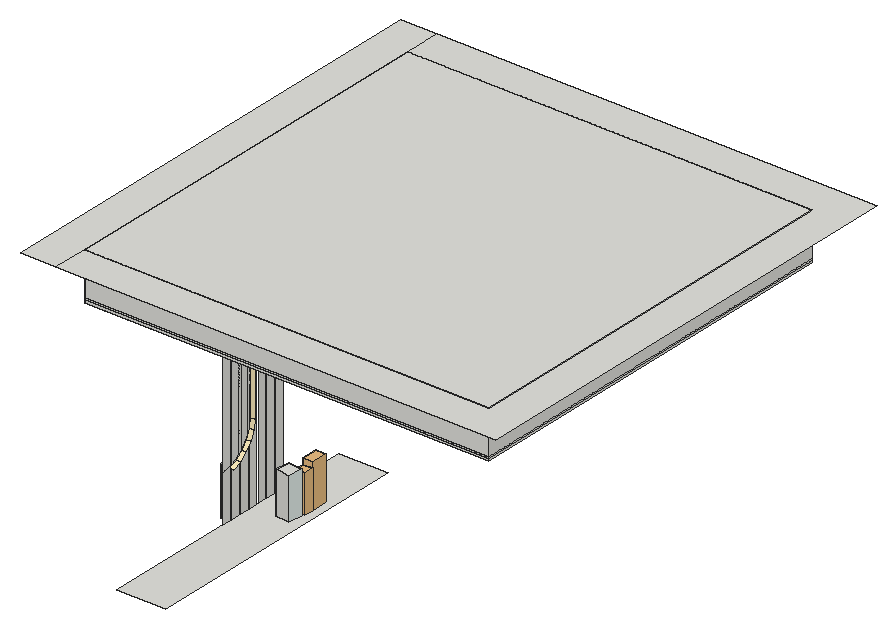
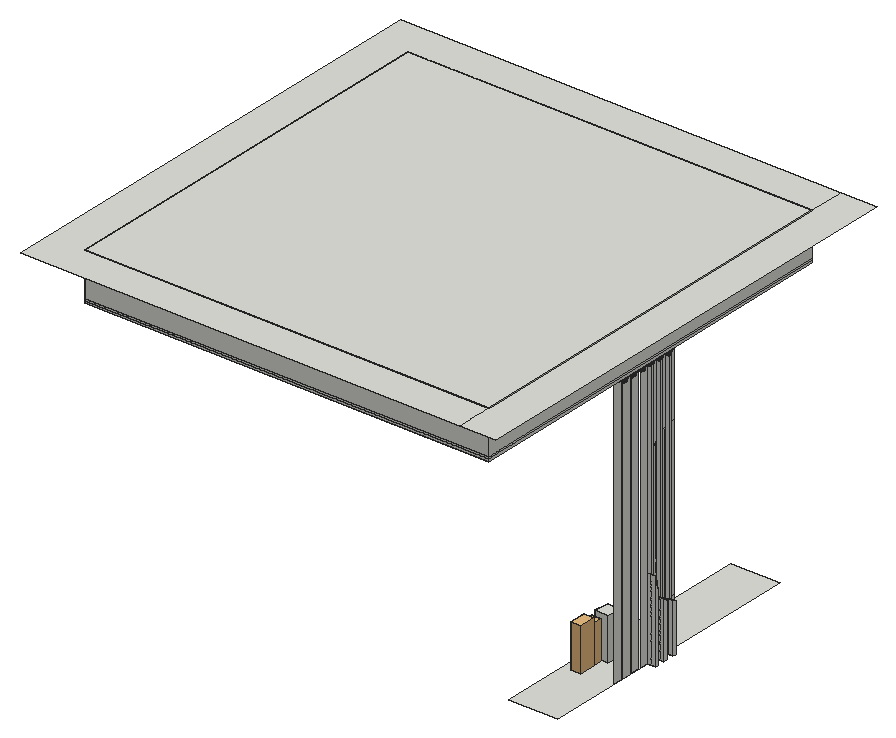
# SketchUp Ruby script. Lengths in inches.
U = 1.inch
M = Sketchup.active_model
def pt(a) = Geom::Point3d.new(a.map { |v| v * U })
def face(e, loops, mat)
  f = e.add_face(loops[0].map { |a| pt(a) })
  loops[1..].each { |l| e.add_face(l.map { |a| pt(a) }).erase! }
  f.material = f.back_material = mat if mat
  f
end
# faces: each face lists its corners as indices into pts; further lists are holes
def faces(e, pts, list, mat = nil) = list.each { |f| face(e, (f[0].is_a?(Array) ? f : [f]).map { |l| l.map { |i| pts[i] } }, mat) }
# xy, xz, yz: faces in a plane at the given z, y or x. An outline is a flat list of corners, or four numbers for a rectangle; further outlines are holes
def ring(l) = l.size == 4 ? [[l[0], l[1]], [l[2], l[1]], [l[2], l[3]], [l[0], l[3]]] : l.each_slice(2).to_a
def flat(e, list, mat, &to3) = list.each { |f| face(e, (f[0].is_a?(Array) ? f : [f]).map { |l| ring(l).map { |u, v| to3.(u, v) } }, mat) }
def xy(e, z, list, mat = nil) = flat(e, list, mat) { |x, y| [x, y, z] }
def xz(e, y, list, mat = nil) = flat(e, list, mat) { |x, z| [x, y, z] }
def yz(e, x, list, mat = nil) = flat(e, list, mat) { |y, z| [x, y, z] }
def lines(e, pts, list) = list.each { |a, b| e.add_line(pt(pts[a]), pt(pts[b])) }
# prism: a flat outline (further loops are holes) pulled along v
def prism(e, loops, v, mat = nil)
  f = face(e, loops, mat); d = Geom::Vector3d.new(v.map { |x| x * U })
  f.pushpull(f.normal.samedirection?(d) ? d.length : -d.length)
end
def box(e, o, s, mat = nil) = prism(e, [[o, [o[0] + s[0], o[1], o[2]], [o[0] + s[0], o[1] + s[1], o[2]], [o[0], o[1] + s[1], o[2]]]], [0, 0, s[2]], mat)
def at(x, y, z, deg = 0) = Geom::Transformation.translation(pt([x, y, z])) * Geom::Transformation.rotation(ORIGIN, Z_AXIS, deg.degrees)
def axes(o, x, y, z) = Geom::Transformation.new([*x, 0, *y, 0, *z, 0, *pt(o).to_a, 1])
def part(name) = M.definitions.add(name)
# library, detail: a bought-in or finely detailed component or shape, given as its bounding box
def library(name, o, s) = part(name).tap { |d| box(d.entities, o, s) }
def detail(e, o, s) = box(e.add_group.entities, o, s)
def put(e, d, t, mat = nil) = e.add_instance(d, t).tap { |i| i.material = mat if mat }
def group(e, t, mat = nil) = e.add_group.tap { |g| g.transformation = t; g.material = mat if mat }.entities
root = M.entities
M.materials.add("Heather_PantShadow").color = [249, 233, 187]
M.materials.add("profumo-muschio-natures-511x511").color = [223, 234, 229]
c1 = part("Component\#12")
xy(c1.entities,0,[[0,0,3.21,3.15]],"profumo-muschio-natures-511x511")
xy(c1.entities,9.32,[[0,0,3.21,3.15]])
xz(c1.entities,0,[[0,0,3.21,9.32]],"profumo-muschio-natures-511x511")
xz(c1.entities,3.15,[[0,0,3.21,9.32]])
yz(c1.entities,0,[[0,0,3.15,9.32]])
yz(c1.entities,3.21,[[0,0,3.15,9.32]])
c2 = library("Toiletry bottle",[0,0,0],[3.45,3.45,11.12])
c3 = library("Toiletry bottle \#2",[0,0,0],[4.22,2.62,10.91])
xy(root,39.466,[[10,18.018,22.25,88.07],[7.875,53.55,10,54.256],[7.875,56.338,10,57.043],[7.875,59.125,10,59.831]])
xy(root,108,[[9,52.455,10,52.564],[9,55.242,10,55.351],[9,58.03,10,58.139],[9,60.817,10,60.926],[9,63.605,10,63.714],
  [9,66.392,10,66.501],[9,69.18,10,69.289]])
xy(root,120,[[0,0,9,120],[9,0,120,0,120,120,9,120,9,111,111,111,111,9,9,9]])
xz(root,53.55,[[7.875,39.466,9,51.606],[9,39.466,10,51.606],[9,51.606,10,106.961]])
xz(root,54.256,[[7.875,39.466,9,51.899],[9,39.466,10,51.899],[9,51.899,10,106.961]])
xz(root,56.338,[[7.875,39.466,9,53.1],[9,39.466,10,53.1],[9,53.1,10,106.961]])
xz(root,57.043,[[7.875,39.466,9,53.642],[9,39.466,10,53.642],[9,53.642,10,106.961]])
xz(root,59.125,[[7.875,39.466,9,56.8],[9,39.466,10,56.8],[9,56.8,10,106.961]])
xz(root,59.831,[[7.875,39.466,9,60.077],[9,39.466,10,60.077],[9,60.077,10,106.961]])
xz(root,59.831,[[10,60.077,11.25,82.153]],"Heather_PantShadow")
yz(root,7.875,[[53.55,39.466,54.256,39.466,54.256,51.899,53.55,51.606],[56.338,39.466,57.043,39.466,57.043,53.642,56.338,53.1],[59.125,39.466,59.831,39.466,59.831,60.077,59.528,57.772,59.125,56.8]])
yz(root,9,[[52.455,108,52.564,108,52.509,108.001],[55.242,108,55.351,108,55.297,108.001],[58.03,108,58.139,108,58.084,108.001],[60.817,108,60.926,108,60.872,108.001],[63.605,108,63.714,108,63.659,108.001],
  [66.392,108,66.501,108,66.447,108.001],[69.18,108,69.289,108,69.234,108.001]])
yz(root,10,[[51.468,39.466,53.55,39.466,53.55,51.606,53.23,51.474,51.468,51.242],[54.256,39.466,56.338,39.466,56.338,53.1,55.378,52.364,54.256,51.899],[57.043,39.466,59.125,39.466,59.125,56.8,58.638,55.624,57.222,53.779,57.043,53.642],[59.831,39.466,61.912,39.466,61.912,106.961,61.911,107.015,61.907,107.069,61.9,107.123,61.89,107.177,61.877,107.23,61.862,107.282,61.843,107.334,61.823,107.384,61.799,107.433,61.773,107.481,61.745,107.528,61.714,107.572,61.681,107.616,61.645,107.657,61.608,107.697,61.568,107.734,61.527,107.769,61.483,107.803,61.439,107.834,61.392,107.862,61.344,107.888,61.295,107.911,61.245,107.932,61.193,107.95,61.141,107.966,61.088,107.979,61.035,107.989,60.981,107.996,60.926,108,60.817,108,60.763,107.996,60.709,107.989,60.655,107.979,60.602,107.966,60.55,107.95,60.499,107.932,60.448,107.911,60.399,107.888,60.351,107.862,60.305,107.834,60.26,107.803,60.217,107.769,60.175,107.734,60.136,107.697,60.098,107.657,60.063,107.616,60.03,107.572,59.999,107.528,59.97,107.481,59.944,107.433,59.921,107.384,59.9,107.334,59.882,107.282,59.866,107.23,59.854,107.177,59.844,107.123,59.837,107.069,59.832,107.015,59.831,106.961],[62.618,39.466,64.7,39.466,64.7,106.961,64.699,107.015,64.694,107.069,64.687,107.123,64.677,107.177,64.665,107.23,64.649,107.282,64.631,107.334,64.61,107.384,64.587,107.433,64.561,107.481,64.532,107.528,64.501,107.572,64.468,107.616,64.433,107.657,64.395,107.697,64.356,107.734,64.314,107.769,64.271,107.803,64.226,107.834,64.18,107.862,64.132,107.888,64.083,107.911,64.032,107.932,63.981,107.95,63.929,107.966,63.876,107.979,63.822,107.989,63.768,107.996,63.714,108,63.605,108,63.55,107.996,63.496,107.989,63.443,107.979,63.39,107.966,63.338,107.95,63.286,107.932,63.236,107.911,63.187,107.888,63.139,107.862,63.092,107.834,63.048,107.803,63.004,107.769,62.963,107.734,62.923,107.697,62.886,107.657,62.85,107.616,62.817,107.572,62.786,107.528,62.758,107.481,62.732,107.433,62.708,107.384,62.6875,107.334,62.669,107.282,62.654,107.23,62.641,107.177,62.631,107.123,62.624,107.069,62.62,107.015,62.618,106.961],
  [65.406,39.466,67.487,39.466,67.487,106.961,67.486,107.015,67.482,107.069,67.475,107.123,67.465,107.177,67.452,107.23,67.437,107.282,67.418,107.334,67.398,107.384,67.374,107.433,67.348,107.481,67.32,107.528,67.289,107.572,67.256,107.616,67.22,107.657,67.183,107.697,67.143,107.734,67.102,107.769,67.058,107.803,67.014,107.834,66.967,107.862,66.919,107.888,66.87,107.911,66.82,107.932,66.768,107.95,66.716,107.966,66.663,107.979,66.61,107.989,66.556,107.996,66.501,108,66.392,108,66.338,107.996,66.284,107.989,66.23,107.979,66.177,107.966,66.125,107.95,66.074,107.932,66.023,107.911,65.974,107.888,65.926,107.862,65.88,107.834,65.835,107.803,65.792,107.769,65.75,107.734,65.711,107.697,65.673,107.657,65.638,107.616,65.605,107.572,65.574,107.528,65.545,107.481,65.519,107.433,65.496,107.384,65.475,107.334,65.457,107.282,65.441,107.23,65.429,107.177,65.419,107.123,65.412,107.069,65.407,107.015,65.406,106.961],[68.193,39.466,70.275,39.466,70.275,106.961,70.274,107.015,70.269,107.069,70.262,107.123,70.252,107.177,70.24,107.23,70.224,107.282,70.206,107.334,70.185,107.384,70.162,107.433,70.136,107.481,70.107,107.528,70.076,107.572,70.043,107.616,70.008,107.657,69.97,107.697,69.931,107.734,69.889,107.769,69.846,107.803,69.801,107.834,69.755,107.862,69.707,107.888,69.658,107.911,69.607,107.932,69.556,107.95,69.504,107.966,69.451,107.979,69.397,107.989,69.343,107.996,69.289,108,69.18,108,69.125,107.996,69.071,107.989,69.018,107.979,68.965,107.966,68.913,107.95,68.861,107.932,68.811,107.911,68.762,107.888,68.714,107.862,68.667,107.834,68.623,107.803,68.579,107.769,68.538,107.734,68.498,107.697,68.461,107.657,68.425,107.616,68.392,107.572,68.361,107.528,68.333,107.481,68.307,107.433,68.283,107.384,68.263,107.334,68.244,107.282,68.229,107.23,68.216,107.177,68.206,107.123,68.199,107.069,68.195,107.015,68.193,106.961],[51.468,51.242,53.23,51.474,53.55,51.606,53.55,90.623,53.23,90.756,51.468,90.988],[53.55,51.606,53.55,90.623,54.256,90.331,54.256,51.899],[54.256,51.899,55.378,52.364,56.338,53.1,56.338,89.13,55.378,89.866,54.256,90.331],
  [56.338,53.1,56.338,89.13,57.043,88.588,57.043,53.642],[57.043,53.642,57.222,53.779,58.638,55.624,59.125,56.8,59.125,85.43,58.638,86.606,57.222,88.451,57.043,88.588],[59.125,56.8,59.125,85.43,59.528,84.458,59.831,82.153,59.831,60.077,59.528,57.772],[59.125,85.43,59.125,106.961,59.124,107.015,59.119,107.069,59.112,107.123,59.102,107.177,59.09,107.23,59.074,107.282,59.056,107.334,59.035,107.384,59.012,107.433,58.986,107.481,58.957,107.528,58.926,107.572,58.893,107.616,58.858,107.657,58.82,107.697,58.781,107.734,58.739,107.769,58.696,107.803,58.651,107.834,58.605,107.862,58.557,107.888,58.508,107.911,58.457,107.932,58.406,107.95,58.354,107.966,58.301,107.979,58.247,107.989,58.193,107.996,58.139,108,58.03,108,57.975,107.996,57.921,107.989,57.868,107.979,57.815,107.966,57.763,107.95,57.711,107.932,57.661,107.911,57.612,107.888,57.564,107.862,57.517,107.834,57.473,107.803,57.429,107.769,57.388,107.734,57.348,107.697,57.311,107.657,57.275,107.616,57.242,107.572,57.211,107.528,57.183,107.481,57.157,107.433,57.133,107.384,57.113,107.334,57.094,107.282,57.079,107.23,57.066,107.177,57.056,107.123,57.049,107.069,57.045,107.015,57.043,106.961,57.043,88.588,57.222,88.451,58.638,86.606],[56.338,89.13,56.338,106.961,56.336,107.015,56.332,107.069,56.325,107.123,56.315,107.177,56.302,107.23,56.287,107.282,56.268,107.334,56.248,107.384,56.224,107.433,56.198,107.481,56.17,107.528,56.139,107.572,56.106,107.616,56.07,107.657,56.033,107.697,55.993,107.734,55.952,107.769,55.908,107.803,55.864,107.834,55.817,107.862,55.769,107.888,55.72,107.911,55.67,107.932,55.618,107.95,55.566,107.966,55.513,107.979,55.46,107.989,55.406,107.996,55.351,108,55.242,108,55.188,107.996,55.134,107.989,55.08,107.979,55.027,107.966,54.975,107.95,54.924,107.932,54.873,107.911,54.824,107.888,54.776,107.862,54.73,107.834,54.685,107.803,54.642,107.769,54.6,107.734,54.561,107.697,54.523,107.657,54.488,107.616,54.455,107.572,54.424,107.528,54.395,107.481,54.369,107.433,54.346,107.384,54.325,107.334,54.307,107.282,54.291,107.23,54.279,107.177,54.269,107.123,54.262,107.069,54.257,107.015,54.256,106.961,54.256,90.331,55.378,89.866],
  [53.55,90.623,53.55,106.961,53.549,107.015,53.544,107.069,53.537,107.123,53.527,107.177,53.515,107.23,53.499,107.282,53.481,107.334,53.46,107.384,53.437,107.433,53.411,107.481,53.382,107.528,53.351,107.572,53.318,107.616,53.283,107.657,53.245,107.697,53.206,107.734,53.164,107.769,53.121,107.803,53.076,107.834,53.03,107.862,52.982,107.888,52.933,107.911,52.882,107.932,52.831,107.95,52.779,107.966,52.726,107.979,52.672,107.989,52.618,107.996,52.564,108,52.455,108,52.4,107.996,52.346,107.989,52.293,107.979,52.24,107.966,52.1875,107.95,52.136,107.932,52.086,107.911,52.037,107.888,51.989,107.862,51.942,107.834,51.898,107.803,51.854,107.769,51.813,107.734,51.773,107.697,51.736,107.657,51.7,107.616,51.667,107.572,51.636,107.528,51.608,107.481,51.582,107.433,51.558,107.384,51.538,107.334,51.519,107.282,51.504,107.23,51.491,107.177,51.481,107.123,51.474,107.069,51.47,107.015,51.468,106.961,51.468,90.988,53.23,90.756]])
p = [[11.25,55.378,52.364],[11.25,53.23,51.474],[10,53.23,51.474],[10,53.55,51.606],[10,54.256,51.899],[10,55.378,52.364],
  [9,53.55,51.606],[7.875,53.55,51.606],[7.875,54.256,51.899],[9,54.256,51.899],[11.25,57.222,53.779],[10,56.338,53.1],
  [10,57.043,53.642],[10,57.222,53.779],[9,56.338,53.1],[7.875,56.338,53.1],[7.875,57.043,53.642],[9,57.043,53.642],
  [11.25,58.638,55.624],[10,58.638,55.624],[11.25,59.528,57.772],[10,59.125,56.8],[10,59.528,57.772],[9,59.125,56.8],
  [7.875,59.125,56.8],[7.875,59.528,57.772],[10,59.831,60.077],[7.875,59.831,60.077],[9,59.831,60.077],[11.25,59.831,60.077],
  [11.25,59.528,84.458],[11.25,59.831,82.153],[10,59.831,82.153],[10,59.528,84.458],[11.25,58.638,86.606],[10,59.125,85.43],
  [10,58.638,86.606],[11.25,57.222,88.451],[10,57.222,88.451],[11.25,55.378,89.866],[10,57.043,88.588],[10,56.338,89.13],
  [10,55.378,89.866],[11.25,53.23,90.756],[10,54.256,90.331],[10,53.55,90.623],[10,53.23,90.756],[9,53.549,107.015],
  [9,53.544,107.069],[10,53.544,107.069],[10,53.549,107.015],[9,53.55,106.961],[10,53.55,106.961],[9,54.257,107.015],
  [9,54.256,106.961],[10,54.256,106.961],[10,54.257,107.015],[9,54.262,107.069],[10,54.262,107.069],[9,56.336,107.015],
  [9,56.332,107.069],[10,56.332,107.069],[10,56.336,107.015],[9,56.338,106.961],[10,56.338,106.961],[9,57.045,107.015],
  [9,57.043,106.961],[10,57.043,106.961],[10,57.045,107.015],[9,57.049,107.069],[10,57.049,107.069],[9,59.124,107.015],
  [9,59.119,107.069],[10,59.119,107.069],[10,59.124,107.015],[9,59.125,106.961],[10,59.125,106.961],[9,59.832,107.015],
  [9,59.831,106.961],[10,59.831,106.961],[10,59.832,107.015],[9,59.837,107.069],[10,59.837,107.069],[9,61.911,107.015],
  [9,61.907,107.069],[10,61.907,107.069],[10,61.911,107.015],[9,61.912,106.961],[10,61.912,106.961],[9,62.62,107.015],
  [9,62.618,106.961],[10,62.618,106.961],[10,62.62,107.015],[9,62.624,107.069],[10,62.624,107.069],[9,64.699,107.015],
  [9,64.694,107.069],[10,64.694,107.069],[10,64.699,107.015],[9,64.7,106.961],[10,64.7,106.961],[9,65.407,107.015],
  [9,65.406,106.961],[10,65.406,106.961],[10,65.407,107.015],[9,65.412,107.069],[10,65.412,107.069],[9,67.486,107.015],
  [9,67.482,107.069],[10,67.482,107.069],[10,67.486,107.015],[9,67.487,106.961],[10,67.487,106.961],[9,68.195,107.015],
  [9,68.193,106.961],[10,68.193,106.961],[10,68.195,107.015],[9,68.199,107.069],[10,68.199,107.069],[9,53.537,107.123],
  [9,53.527,107.177],[10,53.527,107.177],[10,53.537,107.123],[9,54.269,107.123],[10,54.269,107.123],[9,54.279,107.177],
  [10,54.279,107.177],[9,56.325,107.123],[9,56.315,107.177],[10,56.315,107.177],[10,56.325,107.123],[9,57.056,107.123],
  [10,57.056,107.123],[9,57.066,107.177],[10,57.066,107.177],[9,59.112,107.123],[9,59.102,107.177],[10,59.102,107.177],
  [10,59.112,107.123],[9,59.844,107.123],[10,59.844,107.123],[9,59.854,107.177],[10,59.854,107.177],[9,61.9,107.123],
  [9,61.89,107.177],[10,61.89,107.177],[10,61.9,107.123],[9,62.631,107.123],[10,62.631,107.123],[9,62.641,107.177],
  [10,62.641,107.177],[9,64.687,107.123],[9,64.677,107.177],[10,64.677,107.177],[10,64.687,107.123],[9,65.419,107.123],
  [10,65.419,107.123],[9,65.429,107.177],[10,65.429,107.177],[9,67.475,107.123],[9,67.465,107.177],[10,67.465,107.177],
  [10,67.475,107.123],[9,68.206,107.123],[10,68.206,107.123],[9,68.216,107.177],[10,68.216,107.177],[9,53.515,107.23],
  [9,53.499,107.282],[10,53.499,107.282],[10,53.515,107.23],[9,54.291,107.23],[10,54.291,107.23],[9,54.307,107.282],
  [10,54.307,107.282],[9,56.302,107.23],[9,56.287,107.282],[10,56.287,107.282],[10,56.302,107.23],[9,57.079,107.23],
  [10,57.079,107.23],[9,57.094,107.282],[10,57.094,107.282],[9,59.09,107.23],[9,59.074,107.282],[10,59.074,107.282],
  [10,59.09,107.23],[9,59.866,107.23],[10,59.866,107.23],[9,59.882,107.282],[10,59.882,107.282],[9,61.877,107.23],
  [9,61.862,107.282],[10,61.862,107.282],[10,61.877,107.23],[9,62.654,107.23],[10,62.654,107.23],[9,62.669,107.282],
  [10,62.669,107.282],[9,64.665,107.23],[9,64.649,107.282],[10,64.649,107.282],[10,64.665,107.23],[9,65.441,107.23],
  [10,65.441,107.23],[9,65.457,107.282],[10,65.457,107.282],[9,67.452,107.23],[9,67.437,107.282],[10,67.437,107.282],
  [10,67.452,107.23],[9,68.229,107.23],[10,68.229,107.23],[9,68.244,107.282],[10,68.244,107.282],[9,53.481,107.334],
  [9,53.46,107.384],[10,53.46,107.384],[10,53.481,107.334],[9,54.325,107.334],[10,54.325,107.334],[9,54.346,107.384],
  [10,54.346,107.384],[9,56.268,107.334],[9,56.248,107.384],[10,56.248,107.384],[10,56.268,107.334],[9,57.113,107.334],
  [10,57.113,107.334],[9,57.133,107.384],[10,57.133,107.384],[9,59.056,107.334],[9,59.035,107.384],[10,59.035,107.384],
  [10,59.056,107.334],[9,59.9,107.334],[10,59.9,107.334],[9,59.921,107.384],[10,59.921,107.384],[9,61.843,107.334],
  [9,61.823,107.384],[10,61.823,107.384],[10,61.843,107.334],[9,62.6875,107.334],[10,62.6875,107.334],[9,62.708,107.384],
  [10,62.708,107.384],[9,64.631,107.334],[9,64.61,107.384],[10,64.61,107.384],[10,64.631,107.334],[9,65.475,107.334],
  [10,65.475,107.334],[9,65.496,107.384],[10,65.496,107.384],[9,67.418,107.334],[9,67.398,107.384],[10,67.398,107.384],
  [10,67.418,107.334],[9,68.263,107.334],[10,68.263,107.334],[9,68.283,107.384],[10,68.283,107.384],[9,53.437,107.433],
  [9,53.411,107.481],[10,53.411,107.481],[10,53.437,107.433],[9,54.369,107.433],[10,54.369,107.433],[9,54.395,107.481],
  [10,54.395,107.481],[9,56.224,107.433],[9,56.198,107.481],[10,56.198,107.481],[10,56.224,107.433],[9,57.157,107.433],
  [10,57.157,107.433],[9,57.183,107.481],[10,57.183,107.481],[9,59.012,107.433],[9,58.986,107.481],[10,58.986,107.481],
  [10,59.012,107.433],[9,59.944,107.433],[10,59.944,107.433],[9,59.97,107.481],[10,59.97,107.481],[9,61.799,107.433],
  [9,61.773,107.481],[10,61.773,107.481],[10,61.799,107.433],[9,62.732,107.433],[10,62.732,107.433],[9,62.758,107.481],
  [10,62.758,107.481],[9,64.587,107.433],[9,64.561,107.481],[10,64.561,107.481],[10,64.587,107.433],[9,65.519,107.433],
  [10,65.519,107.433],[9,65.545,107.481],[10,65.545,107.481],[9,67.374,107.433],[9,67.348,107.481],[10,67.348,107.481],
  [10,67.374,107.433],[9,68.307,107.433],[10,68.307,107.433],[9,68.333,107.481],[10,68.333,107.481],[9,53.382,107.528],
  [9,53.351,107.572],[10,53.351,107.572],[10,53.382,107.528],[9,54.424,107.528],[10,54.424,107.528],[9,54.455,107.572],
  [10,54.455,107.572],[9,56.17,107.528],[9,56.139,107.572],[10,56.139,107.572],[10,56.17,107.528],[9,57.211,107.528],
  [10,57.211,107.528],[9,57.242,107.572],[10,57.242,107.572],[9,58.957,107.528],[9,58.926,107.572],[10,58.926,107.572],
  [10,58.957,107.528],[9,59.999,107.528],[10,59.999,107.528],[9,60.03,107.572],[10,60.03,107.572],[9,61.745,107.528],
  [9,61.714,107.572],[10,61.714,107.572],[10,61.745,107.528],[9,62.786,107.528],[10,62.786,107.528],[9,62.817,107.572],
  [10,62.817,107.572],[9,64.532,107.528],[9,64.501,107.572],[10,64.501,107.572],[10,64.532,107.528],[9,65.574,107.528],
  [10,65.574,107.528],[9,65.605,107.572],[10,65.605,107.572],[9,67.32,107.528],[9,67.289,107.572],[10,67.289,107.572],
  [10,67.32,107.528],[9,68.361,107.528],[10,68.361,107.528],[9,68.392,107.572],[10,68.392,107.572],[9,53.318,107.616],
  [9,53.283,107.657],[10,53.283,107.657],[10,53.318,107.616],[9,54.488,107.616],[10,54.488,107.616],[9,54.523,107.657],
  [10,54.523,107.657],[9,56.106,107.616],[9,56.07,107.657],[10,56.07,107.657],[10,56.106,107.616],[9,57.275,107.616],
  [10,57.275,107.616],[9,57.311,107.657],[10,57.311,107.657],[9,58.893,107.616],[9,58.858,107.657],[10,58.858,107.657],
  [10,58.893,107.616],[9,60.063,107.616],[10,60.063,107.616],[9,60.098,107.657],[10,60.098,107.657],[9,61.681,107.616],
  [9,61.645,107.657],[10,61.645,107.657],[10,61.681,107.616],[9,62.85,107.616],[10,62.85,107.616],[9,62.886,107.657],
  [10,62.886,107.657],[9,64.468,107.616],[9,64.433,107.657],[10,64.433,107.657],[10,64.468,107.616],[9,65.638,107.616],
  [10,65.638,107.616],[9,65.673,107.657],[10,65.673,107.657],[9,67.256,107.616],[9,67.22,107.657],[10,67.22,107.657],
  [10,67.256,107.616],[9,68.425,107.616],[10,68.425,107.616],[9,68.461,107.657],[10,68.461,107.657],[9,53.206,107.734],
  [9,53.164,107.769],[10,53.164,107.769],[10,53.206,107.734],[9,53.245,107.697],[10,53.245,107.697],[9,54.561,107.697],
  [10,54.561,107.697],[9,54.6,107.734],[10,54.6,107.734],[9,54.642,107.769],[10,54.642,107.769],[9,55.993,107.734],
  [9,55.952,107.769],[10,55.952,107.769],[10,55.993,107.734],[9,56.033,107.697],[10,56.033,107.697],[9,57.348,107.697],
  [10,57.348,107.697],[9,57.388,107.734],[10,57.388,107.734],[9,57.429,107.769],[10,57.429,107.769],[9,58.781,107.734],
  [9,58.739,107.769],[10,58.739,107.769],[10,58.781,107.734],[9,58.82,107.697],[10,58.82,107.697],[9,60.136,107.697],
  [10,60.136,107.697],[9,60.175,107.734],[10,60.175,107.734],[9,60.217,107.769],[10,60.217,107.769],[9,61.568,107.734],
  [9,61.527,107.769],[10,61.527,107.769],[10,61.568,107.734],[9,61.608,107.697],[10,61.608,107.697],[9,62.923,107.697],
  [10,62.923,107.697],[9,62.963,107.734],[10,62.963,107.734],[9,63.004,107.769],[10,63.004,107.769],[9,64.356,107.734],
  [9,64.314,107.769],[10,64.314,107.769],[10,64.356,107.734],[9,64.395,107.697],[10,64.395,107.697],[9,65.711,107.697],
  [10,65.711,107.697],[9,65.75,107.734],[10,65.75,107.734],[9,65.792,107.769],[10,65.792,107.769],[9,67.143,107.734],
  [9,67.102,107.769],[10,67.102,107.769],[10,67.143,107.734],[9,67.183,107.697],[10,67.183,107.697],[9,68.498,107.697],
  [10,68.498,107.697],[9,68.538,107.734],[10,68.538,107.734],[9,68.579,107.769],[10,68.579,107.769],[9,53.076,107.834],
  [9,53.03,107.862],[10,53.03,107.862],[10,53.076,107.834],[9,53.121,107.803],[10,53.121,107.803],[9,54.685,107.803],
  [10,54.685,107.803],[9,54.73,107.834],[10,54.73,107.834],[9,54.776,107.862],[10,54.776,107.862],[9,55.864,107.834],
  [9,55.817,107.862],[10,55.817,107.862],[10,55.864,107.834],[9,55.908,107.803],[10,55.908,107.803],[9,57.473,107.803],
  [10,57.473,107.803],[9,57.517,107.834],[10,57.517,107.834],[9,57.564,107.862],[10,57.564,107.862],[9,58.651,107.834],
  [9,58.605,107.862],[10,58.605,107.862],[10,58.651,107.834],[9,58.696,107.803],[10,58.696,107.803],[9,60.26,107.803],
  [10,60.26,107.803],[9,60.305,107.834],[10,60.305,107.834],[9,60.351,107.862],[10,60.351,107.862],[9,61.439,107.834],
  [9,61.392,107.862],[10,61.392,107.862],[10,61.439,107.834],[9,61.483,107.803],[10,61.483,107.803],[9,63.048,107.803],
  [10,63.048,107.803],[9,63.092,107.834],[10,63.092,107.834],[9,63.139,107.862],[10,63.139,107.862],[9,64.226,107.834],
  [9,64.18,107.862],[10,64.18,107.862],[10,64.226,107.834],[9,64.271,107.803],[10,64.271,107.803],[9,65.835,107.803],
  [10,65.835,107.803],[9,65.88,107.834],[10,65.88,107.834],[9,65.926,107.862],[10,65.926,107.862],[9,67.014,107.834],
  [9,66.967,107.862],[10,66.967,107.862],[10,67.014,107.834],[9,67.058,107.803],[10,67.058,107.803],[9,68.623,107.803],
  [10,68.623,107.803],[9,68.667,107.834],[10,68.667,107.834],[9,68.714,107.862],[10,68.714,107.862],[9,52.086,107.911],
  [9,52.037,107.888],[10,52.037,107.888],[10,52.086,107.911],[9,52.136,107.932],[10,52.136,107.932],[9,52.1875,107.95],
  [10,52.1875,107.95],[9,52.882,107.932],[9,52.831,107.95],[10,52.831,107.95],[10,52.882,107.932],[9,52.933,107.911],
  [10,52.933,107.911],[9,52.982,107.888],[10,52.982,107.888],[9,54.824,107.888],[10,54.824,107.888],[9,54.873,107.911],
  [10,54.873,107.911],[9,54.924,107.932],[10,54.924,107.932],[9,54.975,107.95],[10,54.975,107.95],[9,55.67,107.932],
  [9,55.618,107.95],[10,55.618,107.95],[10,55.67,107.932],[9,55.72,107.911],[10,55.72,107.911],[9,55.769,107.888],
  [10,55.769,107.888],[9,57.612,107.888],[10,57.612,107.888],[9,57.661,107.911],[10,57.661,107.911],[9,57.711,107.932],
  [10,57.711,107.932],[9,57.763,107.95],[10,57.763,107.95],[9,58.457,107.932],[9,58.406,107.95],[10,58.406,107.95],
  [10,58.457,107.932],[9,58.508,107.911],[10,58.508,107.911],[9,58.557,107.888],[10,58.557,107.888],[9,60.399,107.888],
  [10,60.399,107.888],[9,60.448,107.911],[10,60.448,107.911],[9,60.499,107.932],[10,60.499,107.932],[9,60.55,107.95],
  [10,60.55,107.95],[9,61.245,107.932],[9,61.193,107.95],[10,61.193,107.95],[10,61.245,107.932],[9,61.295,107.911],
  [10,61.295,107.911],[9,61.344,107.888],[10,61.344,107.888],[9,63.187,107.888],[10,63.187,107.888],[9,63.236,107.911],
  [10,63.236,107.911],[9,63.286,107.932],[10,63.286,107.932],[9,63.338,107.95],[10,63.338,107.95],[9,64.032,107.932],
  [9,63.981,107.95],[10,63.981,107.95],[10,64.032,107.932],[9,64.083,107.911],[10,64.083,107.911],[9,64.132,107.888],
  [10,64.132,107.888],[9,65.974,107.888],[10,65.974,107.888],[9,66.023,107.911],[10,66.023,107.911],[9,66.074,107.932],
  [10,66.074,107.932],[9,66.125,107.95],[10,66.125,107.95],[9,66.82,107.932],[9,66.768,107.95],[10,66.768,107.95],
  [10,66.82,107.932],[9,66.87,107.911],[10,66.87,107.911],[9,66.919,107.888],[10,66.919,107.888],[9,68.762,107.888],
  [10,68.762,107.888],[9,68.811,107.911],[10,68.811,107.911],[9,68.861,107.932],[10,68.861,107.932],[9,68.913,107.95],
  [10,68.913,107.95],[9,69.607,107.932],[9,69.556,107.95],[10,69.556,107.95],[10,69.607,107.932],[9,69.658,107.911],
  [10,69.658,107.911],[9,69.707,107.888],[10,69.707,107.888],[9,52.24,107.966],[10,52.24,107.966],[9,52.293,107.979],
  [10,52.293,107.979],[9,52.346,107.989],[10,52.346,107.989],[9,52.4,107.996],[10,52.4,107.996],[9,52.455,108],
  [10,52.455,108],[9,52.618,107.996],[9,52.564,108],[10,52.564,108],[10,52.618,107.996],[9,52.672,107.989],
  [10,52.672,107.989],[9,52.726,107.979],[10,52.726,107.979],[9,52.779,107.966],[10,52.779,107.966],[9,55.027,107.966],
  [10,55.027,107.966],[9,55.08,107.979],[10,55.08,107.979],[9,55.134,107.989],[10,55.134,107.989],[9,55.188,107.996],
  [10,55.188,107.996],[9,55.242,108],[10,55.242,108],[9,55.406,107.996],[9,55.351,108],[10,55.351,108],
  [10,55.406,107.996],[9,55.46,107.989],[10,55.46,107.989],[9,55.513,107.979],[10,55.513,107.979],[9,55.566,107.966],
  [10,55.566,107.966],[9,57.815,107.966],[10,57.815,107.966],[9,57.868,107.979],[10,57.868,107.979],[9,57.921,107.989],
  [10,57.921,107.989],[9,57.975,107.996],[10,57.975,107.996],[9,58.03,108],[10,58.03,108],[9,58.193,107.996],
  [9,58.139,108],[10,58.139,108],[10,58.193,107.996],[9,58.247,107.989],[10,58.247,107.989],[9,58.301,107.979],
  [10,58.301,107.979],[9,58.354,107.966],[10,58.354,107.966],[9,60.602,107.966],[10,60.602,107.966],[9,60.655,107.979],
  [10,60.655,107.979],[9,60.709,107.989],[10,60.709,107.989],[9,60.763,107.996],[10,60.763,107.996],[9,60.817,108],
  [10,60.817,108],[9,60.981,107.996],[9,60.926,108],[10,60.926,108],[10,60.981,107.996],[9,61.035,107.989],
  [10,61.035,107.989],[9,61.088,107.979],[10,61.088,107.979],[9,61.141,107.966],[10,61.141,107.966],[9,63.39,107.966],
  [10,63.39,107.966],[9,63.443,107.979],[10,63.443,107.979],[9,63.496,107.989],[10,63.496,107.989],[9,63.55,107.996],
  [10,63.55,107.996],[9,63.605,108],[10,63.605,108],[9,63.768,107.996],[9,63.714,108],[10,63.714,108],
  [10,63.768,107.996],[9,63.822,107.989],[10,63.822,107.989],[9,63.876,107.979],[10,63.876,107.979],[9,63.929,107.966],
  [10,63.929,107.966],[9,66.177,107.966],[10,66.177,107.966],[9,66.23,107.979],[10,66.23,107.979],[9,66.284,107.989],
  [10,66.284,107.989],[9,66.338,107.996],[10,66.338,107.996],[9,66.392,108],[10,66.392,108],[9,66.556,107.996],
  [9,66.501,108],[10,66.501,108],[10,66.556,107.996],[9,66.61,107.989],[10,66.61,107.989],[9,66.663,107.979],
  [10,66.663,107.979],[9,66.716,107.966],[10,66.716,107.966],[9,68.965,107.966],[10,68.965,107.966],[9,69.018,107.979],
  [10,69.018,107.979],[9,69.071,107.989],[10,69.071,107.989],[9,69.125,107.996],[10,69.125,107.996],[9,69.18,108],
  [10,69.18,108],[9,69.343,107.996],[9,69.289,108],[10,69.289,108],[10,69.343,107.996],[9,69.397,107.989],
  [10,69.397,107.989],[9,69.451,107.979],[10,69.451,107.979],[9,69.504,107.966],[10,69.504,107.966]]
faces(root,p,[[0,1,2,3,4,5],[10,0,5,11,12,13],[18,10,13,19],[20,18,19,21,22],[29,20,22,26],[30,31,32,33],[34,30,33,35,36],[37,34,36,38],
  [39,37,38,40,41,42],[43,39,42,44,45,46]],"Heather_PantShadow")
faces(root,p,[[4,3,6,7,8,9],[12,11,14,15,16,17],[22,21,23,24,25],[26,22,25,27,28],[47,48,49,50],[51,47,50,52],[53,54,55,56],[57,53,56,58],
  [59,60,61,62],[63,59,62,64],[65,66,67,68],[69,65,68,70],[71,72,73,74],[75,71,74,76],[77,78,79,80],[81,77,80,82],
  [83,84,85,86],[87,83,86,88],[89,90,91,92],[93,89,92,94],[95,96,97,98],[99,95,98,100],[101,102,103,104],[105,101,104,106],
  [107,108,109,110],[111,107,110,112],[113,114,115,116],[117,113,116,118],[119,120,121,122],[48,119,122,49],[123,57,58,124],[125,123,124,126],
  [127,128,129,130],[60,127,130,61],[131,69,70,132],[133,131,132,134],[135,136,137,138],[72,135,138,73],[139,81,82,140],[141,139,140,142],
  [143,144,145,146],[84,143,146,85],[147,93,94,148],[149,147,148,150],[151,152,153,154],[96,151,154,97],[155,105,106,156],[157,155,156,158],
  [159,160,161,162],[108,159,162,109],[163,117,118,164],[165,163,164,166],[167,168,169,170],[120,167,170,121],[171,125,126,172],[173,171,172,174],
  [175,176,177,178],[128,175,178,129],[179,133,134,180],[181,179,180,182],[183,184,185,186],[136,183,186,137],[187,141,142,188],[189,187,188,190],
  [191,192,193,194],[144,191,194,145],[195,149,150,196],[197,195,196,198],[199,200,201,202],[152,199,202,153],[203,157,158,204],[205,203,204,206],
  [207,208,209,210],[160,207,210,161],[211,165,166,212],[213,211,212,214],[215,216,217,218],[168,215,218,169],[219,173,174,220],[221,219,220,222],
  [223,224,225,226],[176,223,226,177],[227,181,182,228],[229,227,228,230],[231,232,233,234],[184,231,234,185],[235,189,190,236],[237,235,236,238],
  [239,240,241,242],[192,239,242,193],[243,197,198,244],[245,243,244,246],[247,248,249,250],[200,247,250,201],[251,205,206,252],[253,251,252,254],
  [255,256,257,258],[208,255,258,209],[259,213,214,260],[261,259,260,262],[263,264,265,266],[216,263,266,217],[267,221,222,268],[269,267,268,270],
  [271,272,273,274],[224,271,274,225],[275,229,230,276],[277,275,276,278],[279,280,281,282],[232,279,282,233],[283,237,238,284],[285,283,284,286],
  [287,288,289,290],[240,287,290,241],[291,245,246,292],[293,291,292,294],[295,296,297,298],[248,295,298,249],[299,253,254,300],[301,299,300,302],
  [303,304,305,306],[256,303,306,257],[307,261,262,308],[309,307,308,310],[311,312,313,314],[264,311,314,265],[315,269,270,316],[317,315,316,318],
  [319,320,321,322],[272,319,322,273],[323,277,278,324],[325,323,324,326],[327,328,329,330],[280,327,330,281],[331,285,286,332],[333,331,332,334],
  [335,336,337,338],[288,335,338,289],[339,293,294,340],[341,339,340,342],[343,344,345,346],[296,343,346,297],[347,301,302,348],[349,347,348,350],
  [351,352,353,354],[304,351,354,305],[355,309,310,356],[357,355,356,358],[359,360,361,362],[312,359,362,313],[363,317,318,364],[365,363,364,366],
  [367,368,369,370],[320,367,370,321],[371,325,326,372],[373,371,372,374],[375,376,377,378],[328,375,378,329],[379,333,334,380],[381,379,380,382],
  [383,384,385,386],[336,383,386,337],[387,341,342,388],[389,387,388,390],[391,392,393,394],[344,391,394,345],[395,349,350,396],[397,395,396,398],
  [399,400,401,402],[352,399,402,353],[403,357,358,404],[405,403,404,406],[407,408,409,410],[411,407,410,412],[360,411,412,361],[413,365,366,414],
  [415,413,414,416],[417,415,416,418],[419,420,421,422],[423,419,422,424],[368,423,424,369],[425,373,374,426],[427,425,426,428],[429,427,428,430],
  [431,432,433,434],[435,431,434,436],[376,435,436,377],[437,381,382,438],[439,437,438,440],[441,439,440,442],[443,444,445,446],[447,443,446,448],
  [384,447,448,385],[449,389,390,450],[451,449,450,452],[453,451,452,454],[455,456,457,458],[459,455,458,460],[392,459,460,393],[461,397,398,462],
  [463,461,462,464],[465,463,464,466],[467,468,469,470],[471,467,470,472],[400,471,472,401],[473,405,406,474],[475,473,474,476],[477,475,476,478],
  [479,480,481,482],[483,479,482,484],[408,483,484,409],[485,417,418,486],[487,485,486,488],[489,487,488,490],[491,492,493,494],[495,491,494,496],
  [420,495,496,421],[497,429,430,498],[499,497,498,500],[501,499,500,502],[503,504,505,506],[507,503,506,508],[432,507,508,433],[509,441,442,510],
  [511,509,510,512],[513,511,512,514],[515,516,517,518],[519,515,518,520],[444,519,520,445],[521,453,454,522],[523,521,522,524],[525,523,524,526],
  [527,528,529,530],[531,527,530,532],[456,531,532,457],[533,465,466,534],[535,533,534,536],[537,535,536,538],[539,540,541,542],[543,539,542,544],
  [468,543,544,469],[545,477,478,546],[547,545,546,548],[549,547,548,550],[551,552,553,554],[555,551,554,556],[557,555,556,558],[559,560,561,562],
  [563,559,562,564],[565,563,564,566],[480,565,566,481],[567,489,490,568],[569,567,568,570],[571,569,570,572],[573,571,572,574],[575,576,577,578],
  [579,575,578,580],[581,579,580,582],[492,581,582,493],[583,501,502,584],[585,583,584,586],[587,585,586,588],[589,587,588,590],[591,592,593,594],
  [595,591,594,596],[597,595,596,598],[504,597,598,505],[599,513,514,600],[601,599,600,602],[603,601,602,604],[605,603,604,606],[607,608,609,610],
  [611,607,610,612],[613,611,612,614],[516,613,614,517],[615,525,526,616],[617,615,616,618],[619,617,618,620],[621,619,620,622],[623,624,625,626],
  [627,623,626,628],[629,627,628,630],[528,629,630,529],[631,537,538,632],[633,631,632,634],[635,633,634,636],[637,635,636,638],[639,640,641,642],
  [643,639,642,644],[645,643,644,646],[540,645,646,541],[647,549,550,648],[649,647,648,650],[651,649,650,652],[653,651,652,654],[655,656,657,658],
  [659,655,658,660],[661,659,660,662],[663,557,558,664],[665,663,664,666],[667,665,666,668],[669,667,668,670],[671,669,670,672],[673,674,675,676],
  [677,673,676,678],[679,677,678,680],[681,679,680,682],[560,681,682,561],[683,573,574,684],[685,683,684,686],[687,685,686,688],[689,687,688,690],
  [691,689,690,692],[693,694,695,696],[697,693,696,698],[699,697,698,700],[701,699,700,702],[576,701,702,577],[703,589,590,704],[705,703,704,706],
  [707,705,706,708],[709,707,708,710],[711,709,710,712],[713,714,715,716],[717,713,716,718],[719,717,718,720],[721,719,720,722],[592,721,722,593],
  [723,605,606,724],[725,723,724,726],[727,725,726,728],[729,727,728,730],[731,729,730,732],[733,734,735,736],[737,733,736,738],[739,737,738,740],
  [741,739,740,742],[608,741,742,609],[743,621,622,744],[745,743,744,746],[747,745,746,748],[749,747,748,750],[751,749,750,752],[753,754,755,756],
  [757,753,756,758],[759,757,758,760],[761,759,760,762],[624,761,762,625],[763,637,638,764],[765,763,764,766],[767,765,766,768],[769,767,768,770],
  [771,769,770,772],[773,774,775,776],[777,773,776,778],[779,777,778,780],[781,779,780,782],[640,781,782,641],[783,653,654,784],[785,783,784,786],
  [787,785,786,788],[789,787,788,790],[791,789,790,792],[793,794,795,796],[797,793,796,798],[799,797,798,800],[801,799,800,802],[656,801,802,657]])
g1 = group(root,at(9,9,120))
xy(g1,-12,[[[0,0,102,102],[24,24,78,78]],[28,28,74,74]])
xy(g1,-11.5,[[[0,0,102,102],[23,23,79,79]],[23,23,24,78],[24,23,79,24],[78,24,79,78],[23,78,79,79]])
xy(g1,-11,[[[0,0,102,102],[23,23,79,79]],[[23,23,79,79],[28,28,74,74]]])
xy(g1,0,[[0,0,102,102]])
xz(g1,0,[[0,-12,102,-11.5],[0,-11.5,102,-11],[0,-11,102,0]])
xz(g1,23,[[23,-11.5,79,-11]])
xz(g1,24,[[24,-12,78,-11.5]])
xz(g1,28,[[28,-12,74,-11]])
xz(g1,74,[[28,-12,74,-11]])
xz(g1,78,[[24,-12,78,-11.5]])
xz(g1,79,[[23,-11.5,79,-11]])
xz(g1,102,[[0,-12,102,-11.5],[0,-11.5,102,-11],[0,-11,102,0]])
yz(g1,0,[[0,-12,102,-11.5],[0,-11.5,102,-11],[0,-11,102,0]])
yz(g1,23,[[23,-11.5,79,-11]])
yz(g1,24,[[24,-12,78,-11.5]])
yz(g1,28,[[28,-12,74,-11]])
yz(g1,74,[[28,-12,74,-11]])
yz(g1,78,[[24,-12,78,-11.5]])
yz(g1,79,[[23,-11.5,79,-11]])
yz(g1,102,[[0,-12,102,-11.5],[0,-11.5,102,-11],[0,-11,102,0]])
put(root,c1,axes([19.44,60.38,39.47],[0.12596,1.12296,0],[-1.12296,0.12596,0],[0,0,1.13]))
put(root,c2,axes([20.1875,64.61,39.47],[0,0.69,0],[-0.69,0,0],[0,0,0.85643]))
put(root,c3,at(20.1875,67,39.47,90))
